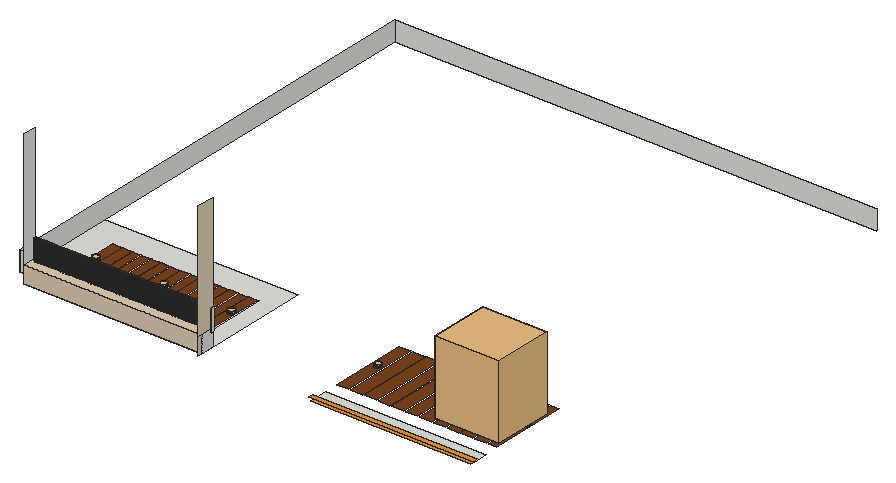
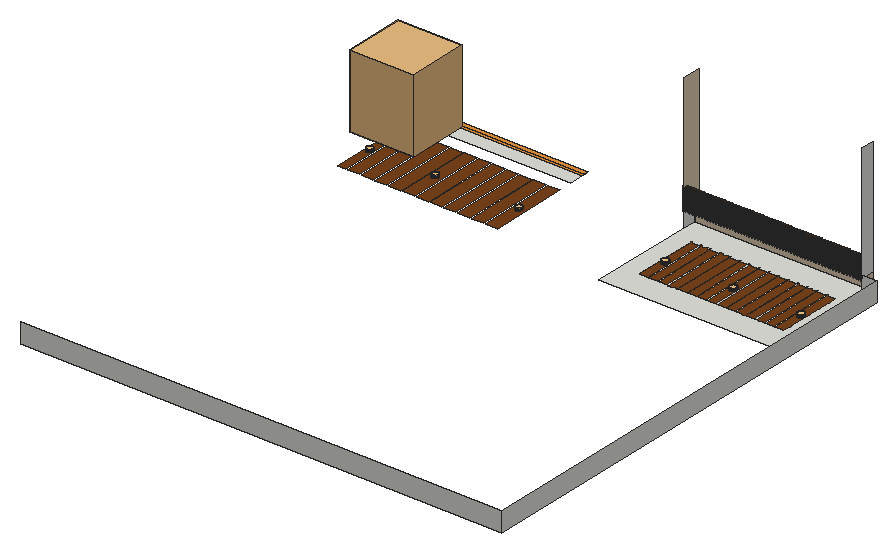
# SketchUp Ruby script. Lengths in inches.
U = 1.inch
M = Sketchup.active_model
def pt(a) = Geom::Point3d.new(a.map { |v| v * U })
def face(e, loops, mat)
  f = e.add_face(loops[0].map { |a| pt(a) })
  loops[1..].each { |l| e.add_face(l.map { |a| pt(a) }).erase! }
  f.material = f.back_material = mat if mat
  f
end
# faces: each face lists its corners as indices into pts; further lists are holes
def faces(e, pts, list, mat = nil) = list.each { |f| face(e, (f[0].is_a?(Array) ? f : [f]).map { |l| l.map { |i| pts[i] } }, mat) }
# xy, xz, yz: faces in a plane at the given z, y or x. An outline is a flat list of corners, or four numbers for a rectangle; further outlines are holes
def ring(l) = l.size == 4 ? [[l[0], l[1]], [l[2], l[1]], [l[2], l[3]], [l[0], l[3]]] : l.each_slice(2).to_a
def flat(e, list, mat, &to3) = list.each { |f| face(e, (f[0].is_a?(Array) ? f : [f]).map { |l| ring(l).map { |u, v| to3.(u, v) } }, mat) }
def xy(e, z, list, mat = nil) = flat(e, list, mat) { |x, y| [x, y, z] }
def xz(e, y, list, mat = nil) = flat(e, list, mat) { |x, z| [x, y, z] }
def yz(e, x, list, mat = nil) = flat(e, list, mat) { |y, z| [x, y, z] }
def lines(e, pts, list) = list.each { |a, b| e.add_line(pt(pts[a]), pt(pts[b])) }
# prism: a flat outline (further loops are holes) pulled along v
def prism(e, loops, v, mat = nil)
  f = face(e, loops, mat); d = Geom::Vector3d.new(v.map { |x| x * U })
  f.pushpull(f.normal.samedirection?(d) ? d.length : -d.length)
end
def box(e, o, s, mat = nil) = prism(e, [[o, [o[0] + s[0], o[1], o[2]], [o[0] + s[0], o[1] + s[1], o[2]], [o[0], o[1] + s[1], o[2]]]], [0, 0, s[2]], mat)
def at(x, y, z, deg = 0) = Geom::Transformation.translation(pt([x, y, z])) * Geom::Transformation.rotation(ORIGIN, Z_AXIS, deg.degrees)
def axes(o, x, y, z) = Geom::Transformation.new([*x, 0, *y, 0, *z, 0, *pt(o).to_a, 1])
def part(name) = M.definitions.add(name)
# library, detail: a bought-in or finely detailed component or shape, given as its bounding box
def library(name, o, s) = part(name).tap { |d| box(d.entities, o, s) }
def detail(e, o, s) = box(e.add_group.entities, o, s)
def put(e, d, t, mat = nil) = e.add_instance(d, t).tap { |i| i.material = mat if mat }
def group(e, t, mat = nil) = e.add_group.tap { |g| g.transformation = t; g.material = mat if mat }.entities
root = M.entities
M.materials.add("Generic\#1").color = [121, 68, 27]
M.materials.add("Generic\#2").color = [245, 199, 133]
M.materials.add("Generic\#4").color = [232, 149, 60]
M.materials.add("Generic\#6").color = [223, 205, 179]
c1 = library("Flora+17",[-57.52,158.6,-38.64],[66.99,62.88,77.28])
c2 = part("Group\#9")
xy(c2.entities,22.76,[[0,0,2,3]])
xz(c2.entities,0,[[0,0,2,22.76]])
yz(c2.entities,0,[[0,0,3,22.76]])
yz(c2.entities,2,[[0,0,3,22.76]])
xy(root,401.75,[[323.78,39.375,491.8125,54.5625],[[17.125,41,204.09,41,204.09,166.1875,2.3125,166.1875,2.3125,54.5625,17.125,54.5625],[32.72,68.9375,185.53,138.25]],[41.97,68.9375,42.91,138.25],[52.16,68.9375,53.09,138.25],[62.34,68.9375,63.28,138.25],
  [72.53,68.9375,73.47,138.25],[82.72,68.9375,83.66,138.25],[92.91,68.9375,93.84,138.25],[103.09,68.9375,104.03,138.25],[113.28,68.9375,114.22,138.25],
  [123.47,68.9375,124.41,138.25],[133.66,68.9375,134.59,138.25],[143.84,68.9375,144.78,138.25],[154.03,68.9375,154.97,138.25],[164.22,68.9375,165.16,138.25],
  [174.41,68.9375,175.34,138.25],[184.59,68.9375,185.53,138.25]])
xy(root,401.75,[[[32.72,68.9375,41.97,138.25],[37.48,106.29,38.4,106.47,39.23,106.87,39.93,107.48,40.46,108.25,40.76,109.13,40.83,110.06,40.65,110.97,40.24,111.81,39.63,112.51,38.86,113.03,37.98,113.34,37.06,113.4,36.14,113.23,35.31,112.82,34.6,112.21,34.08,111.44,33.78,110.5625,33.71,109.63,33.89,108.72,34.3,107.88,34.91,107.18,35.68,106.66,36.55,106.36]],[42.91,68.9375,52.16,138.25],[53.09,68.9375,62.34,138.25],[63.28,68.9375,72.53,138.25],[73.47,68.9375,82.72,138.25],
  [83.66,68.9375,92.91,138.25],[93.84,68.9375,103.09,138.25],[[104.03,68.9375,113.28,138.25],[108.73,106.29,109.65,106.47,110.48,106.87,111.18,107.48,111.71,108.25,112.01,109.13,112.08,110.06,111.9,110.97,111.49,111.81,110.88,112.51,110.11,113.03,109.23,113.34,108.31,113.4,107.39,113.23,106.56,112.82,105.85,112.21,105.33,111.44,105.03,110.5625,104.96,109.63,105.14,108.72,105.55,107.88,106.16,107.18,106.93,106.66,107.8,106.36]],[114.22,68.9375,123.47,138.25],[124.41,68.9375,133.66,138.25],
  [134.59,68.9375,143.84,138.25],[144.78,68.9375,154.03,138.25],[154.97,68.9375,164.22,138.25],[165.16,68.9375,174.41,138.25],[[175.34,68.9375,184.59,138.25],[180.17,106.29,181.08,106.47,181.92,106.87,182.62,107.48,183.14,108.25,183.45,109.13,183.51,110.06,183.34,110.97,182.93,111.81,182.32,112.51,181.55,113.03,180.67,113.34,179.74,113.4,178.83,113.23,177.99,112.82,177.29,112.21,176.77,111.44,176.47,110.5625,176.4,109.63,176.58,108.72,176.98,107.88,177.59,107.18,178.36,106.66,179.24,106.36]],
  [[323.03,69.49,335.53,151.25],[329.74,111.47,330.6,111.58,331.4,111.91,332.08,112.4375,332.61,113.125,332.94,113.92,333.05,114.78,332.94,115.64,332.61,116.4375,332.08,117.12,331.4,117.65,330.6,117.98,329.74,118.09,328.88,117.98,328.08,117.65,327.4,117.12,326.87,116.4375,326.54,115.64,326.43,114.78,326.54,113.92,326.87,113.125,327.4,112.4375,328.08,111.91,328.88,111.58]],[337.53,69.49,350.03,151.25],[352.03,69.49,364.53,151.25],[366.53,69.49,379.03,151.25],[381.03,69.49,393.53,151.25],
  [395.53,69.49,408.03,151.25],[[410.03,69.49,422.53,151.25],[417.49,111.47,418.35,111.58,419.15,111.91,419.83,112.4375,420.36,113.125,420.69,113.92,420.8,114.78,420.69,115.64,420.36,116.4375,419.83,117.12,419.15,117.65,418.35,117.98,417.49,118.09,416.63,117.98,415.83,117.65,415.15,117.12,414.62,116.4375,414.29,115.64,414.18,114.78,414.29,113.92,414.62,113.125,415.15,112.4375,415.83,111.91,416.63,111.58]],[424.53,69.49,437.03,151.25],[439.03,69.49,451.53,151.25],[453.53,69.49,466.03,151.25],
  [468.03,69.49,480.53,151.25],[[482.53,69.49,490.94,151.25],[486.8,111.47,487.66,111.58,488.46,111.91,489.15,112.4375,489.67,113.125,490,113.92,490.12,114.78,490,115.64,489.67,116.4375,489.15,117.12,488.46,117.65,487.66,117.98,486.8,118.09,485.95,117.98,485.15,117.65,484.46,117.12,483.93,116.4375,483.6,115.64,483.49,114.78,483.6,113.92,483.93,113.125,484.46,112.4375,485.15,111.91,485.95,111.58]]],"Generic\#1")
xy(root,401.75,[[323.78,34.75,491.8125,39.375]],"Generic\#4")
xy(root,404.3125,[[37.48,106.29,36.55,106.36,35.68,106.66,34.91,107.18,34.3,107.88,33.89,108.72,33.71,109.63,33.78,110.5625,34.08,111.44,34.6,112.21,35.31,112.82,36.14,113.23,37.06,113.4,37.98,113.34,38.86,113.03,39.63,112.51,40.24,111.81,40.65,110.97,40.83,110.06,40.76,109.13,40.46,108.25,39.93,107.48,39.23,106.87,38.4,106.47],[108.73,106.29,107.8,106.36,106.93,106.66,106.16,107.18,105.55,107.88,105.14,108.72,104.96,109.63,105.03,110.5625,105.33,111.44,105.85,112.21,106.56,112.82,107.39,113.23,108.31,113.4,109.23,113.34,110.11,113.03,110.88,112.51,111.49,111.81,111.9,110.97,112.08,110.06,112.01,109.13,111.71,108.25,111.18,107.48,110.48,106.87,109.65,106.47],[180.17,106.29,179.24,106.36,178.36,106.66,177.59,107.18,176.98,107.88,176.58,108.72,176.4,109.63,176.47,110.5625,176.77,111.44,177.29,112.21,177.99,112.82,178.83,113.23,179.74,113.4,180.67,113.34,181.55,113.03,182.32,112.51,182.93,111.81,183.34,110.97,183.51,110.06,183.45,109.13,183.14,108.25,182.62,107.48,181.92,106.87,181.08,106.47],[329.74,111.47,328.88,111.58,328.08,111.91,327.4,112.4375,326.87,113.125,326.54,113.92,326.43,114.78,326.54,115.64,326.87,116.4375,327.4,117.12,328.08,117.65,328.88,117.98,329.74,118.09,330.6,117.98,331.4,117.65,332.08,117.12,332.61,116.4375,332.94,115.64,333.05,114.78,332.94,113.92,332.61,113.125,332.08,112.4375,331.4,111.91,330.6,111.58],[417.49,111.47,416.63,111.58,415.83,111.91,415.15,112.4375,414.62,113.125,414.29,113.92,414.18,114.78,414.29,115.64,414.62,116.4375,415.15,117.12,415.83,117.65,416.63,117.98,417.49,118.09,418.35,117.98,419.15,117.65,419.83,117.12,420.36,116.4375,420.69,115.64,420.8,114.78,420.69,113.92,420.36,113.125,419.83,112.4375,419.15,111.91,418.35,111.58],
  [486.8,111.47,485.95,111.58,485.15,111.91,484.46,112.4375,483.93,113.125,483.6,113.92,483.49,114.78,483.6,115.64,483.93,116.4375,484.46,117.12,485.15,117.65,485.95,117.98,486.8,118.09,487.66,117.98,488.46,117.65,489.15,117.12,489.67,116.4375,490,115.64,490.12,114.78,490,113.92,489.67,113.125,489.15,112.4375,488.46,111.91,487.66,111.58]],"Generic\#2")
xy(root,404.6875,[[321.31,34.75,494.1875,39.375]],"Generic\#4")
xy(root,419.625,[[17.125,41,204.09,54.5625]],"Generic\#6")
xz(root,41,[[17.125,401.75,204.09,419.625]],"Generic\#6")
xz(root,54.5625,[[2.3125,401.75,17.125,422.625],[17.125,419.625,204.09,440.1875]])
xz(root,546.8125,[[2.3125,401.75,507.875,422.625]])
yz(root,2.3125,[[54.5625,401.75,546.8125,422.625]])
yz(root,17.125,[[41,419.625,54.5625,542.625]])
yz(root,204.09,[[41,401.75,54.5625,419.625]])
yz(root,204.09,[[35.5625,401.75,41,419.625],[35.5625,419.625,54.5625,542.625]],"Generic\#6")
p = [[37.48,106.29,401.75],[36.55,106.36,401.75],[36.55,106.36,404.3125],[37.48,106.29,404.3125],[38.4,106.47,401.75],[38.4,106.47,404.3125],
  [108.73,106.29,401.75],[107.8,106.36,401.75],[107.8,106.36,404.3125],[108.73,106.29,404.3125],[109.65,106.47,401.75],[109.65,106.47,404.3125],
  [180.17,106.29,401.75],[179.24,106.36,401.75],[179.24,106.36,404.3125],[180.17,106.29,404.3125],[181.08,106.47,401.75],[181.08,106.47,404.3125],
  [35.68,106.66,401.75],[35.68,106.66,404.3125],[106.93,106.66,401.75],[106.93,106.66,404.3125],[178.36,106.66,401.75],[178.36,106.66,404.3125],
  [39.23,106.87,401.75],[39.23,106.87,404.3125],[110.48,106.87,401.75],[110.48,106.87,404.3125],[181.92,106.87,401.75],[181.92,106.87,404.3125],
  [34.91,107.18,401.75],[34.91,107.18,404.3125],[106.16,107.18,401.75],[106.16,107.18,404.3125],[177.59,107.18,401.75],[177.59,107.18,404.3125],
  [39.93,107.48,401.75],[39.93,107.48,404.3125],[111.18,107.48,401.75],[111.18,107.48,404.3125],[182.62,107.48,401.75],[182.62,107.48,404.3125],
  [34.3,107.88,401.75],[34.3,107.88,404.3125],[105.55,107.88,401.75],[105.55,107.88,404.3125],[176.98,107.88,401.75],[176.98,107.88,404.3125],
  [40.46,108.25,401.75],[40.46,108.25,404.3125],[111.71,108.25,401.75],[111.71,108.25,404.3125],[183.14,108.25,401.75],[183.14,108.25,404.3125],
  [33.89,108.72,401.75],[33.89,108.72,404.3125],[105.14,108.72,401.75],[105.14,108.72,404.3125],[176.58,108.72,401.75],[176.58,108.72,404.3125],
  [40.76,109.13,401.75],[40.76,109.13,404.3125],[112.01,109.13,401.75],[112.01,109.13,404.3125],[183.45,109.13,401.75],[183.45,109.13,404.3125],
  [33.71,109.63,401.75],[33.71,109.63,404.3125],[104.96,109.63,401.75],[104.96,109.63,404.3125],[176.4,109.63,401.75],[176.4,109.63,404.3125],
  [40.83,110.06,401.75],[40.83,110.06,404.3125],[112.08,110.06,401.75],[112.08,110.06,404.3125],[183.51,110.06,401.75],[183.51,110.06,404.3125],
  [33.78,110.5625,401.75],[33.78,110.5625,404.3125],[105.03,110.5625,401.75],[105.03,110.5625,404.3125],[176.47,110.5625,401.75],[176.47,110.5625,404.3125],
  [40.65,110.97,401.75],[40.65,110.97,404.3125],[111.9,110.97,401.75],[111.9,110.97,404.3125],[183.34,110.97,401.75],[183.34,110.97,404.3125],
  [34.08,111.44,401.75],[34.08,111.44,404.3125],[105.33,111.44,401.75],[105.33,111.44,404.3125],[176.77,111.44,401.75],[176.77,111.44,404.3125],
  [40.24,111.81,401.75],[40.24,111.81,404.3125],[111.49,111.81,401.75],[111.49,111.81,404.3125],[182.93,111.81,401.75],[182.93,111.81,404.3125],
  [34.6,112.21,401.75],[34.6,112.21,404.3125],[105.85,112.21,401.75],[105.85,112.21,404.3125],[177.29,112.21,401.75],[177.29,112.21,404.3125],
  [329.74,111.47,401.75],[328.88,111.58,401.75],[328.88,111.58,404.3125],[329.74,111.47,404.3125],[330.6,111.58,401.75],[330.6,111.58,404.3125],
  [417.49,111.47,401.75],[416.63,111.58,401.75],[416.63,111.58,404.3125],[417.49,111.47,404.3125],[418.35,111.58,401.75],[418.35,111.58,404.3125],
  [486.8,111.47,401.75],[485.95,111.58,401.75],[485.95,111.58,404.3125],[486.8,111.47,404.3125],[487.66,111.58,401.75],[487.66,111.58,404.3125],
  [328.08,111.91,401.75],[328.08,111.91,404.3125],[331.4,111.91,401.75],[331.4,111.91,404.3125],[415.83,111.91,401.75],[415.83,111.91,404.3125],
  [419.15,111.91,401.75],[419.15,111.91,404.3125],[485.15,111.91,401.75],[485.15,111.91,404.3125],[488.46,111.91,401.75],[488.46,111.91,404.3125],
  [39.63,112.51,401.75],[39.63,112.51,404.3125],[110.88,112.51,401.75],[110.88,112.51,404.3125],[182.32,112.51,401.75],[182.32,112.51,404.3125],
  [327.4,112.4375,401.75],[327.4,112.4375,404.3125],[332.08,112.4375,401.75],[332.08,112.4375,404.3125],[415.15,112.4375,401.75],[415.15,112.4375,404.3125],
  [419.83,112.4375,401.75],[419.83,112.4375,404.3125],[484.46,112.4375,401.75],[484.46,112.4375,404.3125],[489.15,112.4375,401.75],[489.15,112.4375,404.3125],
  [35.31,112.82,401.75],[35.31,112.82,404.3125],[106.56,112.82,401.75],[106.56,112.82,404.3125],[177.99,112.82,401.75],[177.99,112.82,404.3125],
  [326.87,113.125,401.75],[326.87,113.125,404.3125],[332.61,113.125,401.75],[332.61,113.125,404.3125],[414.62,113.125,401.75],[414.62,113.125,404.3125],
  [420.36,113.125,401.75],[420.36,113.125,404.3125],[483.93,113.125,401.75],[483.93,113.125,404.3125],[489.67,113.125,401.75],[489.67,113.125,404.3125],
  [38.86,113.03,401.75],[38.86,113.03,404.3125],[110.11,113.03,401.75],[110.11,113.03,404.3125],[181.55,113.03,401.75],[181.55,113.03,404.3125],
  [36.14,113.23,401.75],[36.14,113.23,404.3125],[107.39,113.23,401.75],[107.39,113.23,404.3125],[178.83,113.23,401.75],[178.83,113.23,404.3125],
  [37.98,113.34,401.75],[37.98,113.34,404.3125],[109.23,113.34,401.75],[109.23,113.34,404.3125],[180.67,113.34,401.75],[180.67,113.34,404.3125],
  [326.54,113.92,401.75],[326.54,113.92,404.3125],[332.94,113.92,401.75],[332.94,113.92,404.3125],[414.29,113.92,401.75],[414.29,113.92,404.3125],
  [420.69,113.92,401.75],[420.69,113.92,404.3125],[483.6,113.92,401.75],[483.6,113.92,404.3125],[490,113.92,401.75],[490,113.92,404.3125],
  [37.06,113.4,401.75],[37.06,113.4,404.3125],[108.31,113.4,401.75],[108.31,113.4,404.3125],[179.74,113.4,401.75],[179.74,113.4,404.3125],
  [326.43,114.78,401.75],[326.43,114.78,404.3125],[333.05,114.78,401.75],[333.05,114.78,404.3125],[414.18,114.78,401.75],[414.18,114.78,404.3125],
  [420.8,114.78,401.75],[420.8,114.78,404.3125],[483.49,114.78,401.75],[483.49,114.78,404.3125],[490.12,114.78,401.75],[490.12,114.78,404.3125],
  [326.54,115.64,401.75],[326.54,115.64,404.3125],[332.94,115.64,401.75],[332.94,115.64,404.3125],[414.29,115.64,401.75],[414.29,115.64,404.3125],
  [420.69,115.64,401.75],[420.69,115.64,404.3125],[483.6,115.64,401.75],[483.6,115.64,404.3125],[490,115.64,401.75],[490,115.64,404.3125],
  [326.87,116.4375,401.75],[326.87,116.4375,404.3125],[332.61,116.4375,401.75],[332.61,116.4375,404.3125],[414.62,116.4375,401.75],[414.62,116.4375,404.3125],
  [420.36,116.4375,401.75],[420.36,116.4375,404.3125],[483.93,116.4375,401.75],[483.93,116.4375,404.3125],[489.67,116.4375,401.75],[489.67,116.4375,404.3125],
  [327.4,117.12,401.75],[327.4,117.12,404.3125],[332.08,117.12,401.75],[332.08,117.12,404.3125],[415.15,117.12,401.75],[415.15,117.12,404.3125],
  [419.83,117.12,401.75],[419.83,117.12,404.3125],[484.46,117.12,401.75],[484.46,117.12,404.3125],[489.15,117.12,401.75],[489.15,117.12,404.3125],
  [328.08,117.65,401.75],[328.08,117.65,404.3125],[331.4,117.65,401.75],[331.4,117.65,404.3125],[415.83,117.65,401.75],[415.83,117.65,404.3125],
  [419.15,117.65,401.75],[419.15,117.65,404.3125],[485.15,117.65,401.75],[485.15,117.65,404.3125],[488.46,117.65,401.75],[488.46,117.65,404.3125],
  [328.88,117.98,401.75],[328.88,117.98,404.3125],[330.6,117.98,401.75],[330.6,117.98,404.3125],[416.63,117.98,401.75],[416.63,117.98,404.3125],
  [418.35,117.98,401.75],[418.35,117.98,404.3125],[485.95,117.98,401.75],[485.95,117.98,404.3125],[487.66,117.98,401.75],[487.66,117.98,404.3125],
  [329.74,118.09,401.75],[329.74,118.09,404.3125],[417.49,118.09,401.75],[417.49,118.09,404.3125],[486.8,118.09,401.75],[486.8,118.09,404.3125],
  [32.72,68.9375,401.75],[31.78,68.9375,401.75],[31.78,138.25,401.75],[30.25,68.9375,401.75],[323.78,39.375,404.6875],[323.78,39.375,401.75]]
faces(root,p,[[0,1,2,3],[4,0,3,5],[6,7,8,9],[10,6,9,11],[12,13,14,15],[16,12,15,17],[1,18,19,2],[7,20,21,8],
  [13,22,23,14],[24,4,5,25],[26,10,11,27],[28,16,17,29],[18,30,31,19],[20,32,33,21],[22,34,35,23],[36,24,25,37],
  [38,26,27,39],[40,28,29,41],[30,42,43,31],[32,44,45,33],[34,46,47,35],[48,36,37,49],[50,38,39,51],[52,40,41,53],
  [42,54,55,43],[44,56,57,45],[46,58,59,47],[60,48,49,61],[62,50,51,63],[64,52,53,65],[54,66,67,55],[56,68,69,57],
  [58,70,71,59],[72,60,61,73],[74,62,63,75],[76,64,65,77],[66,78,79,67],[68,80,81,69],[70,82,83,71],[84,72,73,85],
  [86,74,75,87],[88,76,77,89],[78,90,91,79],[80,92,93,81],[82,94,95,83],[96,84,85,97],[98,86,87,99],[100,88,89,101],
  [90,102,103,91],[92,104,105,93],[94,106,107,95],[108,109,110,111],[112,108,111,113],[114,115,116,117],[118,114,117,119],[120,121,122,123],
  [124,120,123,125],[109,126,127,110],[128,112,113,129],[115,130,131,116],[132,118,119,133],[121,134,135,122],[136,124,125,137],[138,96,97,139],
  [140,98,99,141],[142,100,101,143],[126,144,145,127],[146,128,129,147],[130,148,149,131],[150,132,133,151],[134,152,153,135],[154,136,137,155],
  [102,156,157,103],[104,158,159,105],[106,160,161,107],[144,162,163,145],[164,146,147,165],[148,166,167,149],[168,150,151,169],[152,170,171,153],
  [172,154,155,173],[174,138,139,175],[176,140,141,177],[178,142,143,179],[156,180,181,157],[158,182,183,159],[160,184,185,161],[186,174,175,187],
  [188,176,177,189],[190,178,179,191],[162,192,193,163],[194,164,165,195],[166,196,197,167],[198,168,169,199],[170,200,201,171],[202,172,173,203],
  [180,204,205,181],[182,206,207,183],[184,208,209,185],[204,186,187,205],[206,188,189,207],[208,190,191,209],[192,210,211,193],[212,194,195,213],
  [196,214,215,197],[216,198,199,217],[200,218,219,201],[220,202,203,221],[210,222,223,211],[224,212,213,225],[214,226,227,215],[228,216,217,229],
  [218,230,231,219],[232,220,221,233],[222,234,235,223],[236,224,225,237],[226,238,239,227],[240,228,229,241],[230,242,243,231],[244,232,233,245],
  [234,246,247,235],[248,236,237,249],[238,250,251,239],[252,240,241,253],[242,254,255,243],[256,244,245,257],[246,258,259,247],[260,248,249,261],
  [250,262,263,251],[264,252,253,265],[254,266,267,255],[268,256,257,269],[258,270,271,259],[272,260,261,273],[262,274,275,263],[276,264,265,277],
  [266,278,279,267],[280,268,269,281],[270,282,283,271],[282,272,273,283],[274,284,285,275],[284,276,277,285],[278,286,287,279],[286,280,281,287]],"Generic\#2")
lines(root,p,[[288,289],[290,289],[289,291],[292,293]])
put(root,c1,at(493.76,-102.17,454.31))
put(root,c2,at(18.375,51.5625,417.43),"Generic\#1")
put(root,c2,at(21.3125,51.5625,417.43),"Generic\#1")
put(root,c2,at(24.25,51.5625,417.43),"Generic\#1")
put(root,c2,at(27.1875,51.5625,417.43),"Generic\#1")
put(root,c2,at(30.125,51.5625,417.43),"Generic\#1")
put(root,c2,at(33.0625,51.5625,417.43),"Generic\#1")
put(root,c2,at(36,51.5625,417.43),"Generic\#1")
put(root,c2,at(38.9375,51.5625,417.43),"Generic\#1")
put(root,c2,at(41.875,51.5625,417.43),"Generic\#1")
put(root,c2,at(44.8125,51.5625,417.43),"Generic\#1")
put(root,c2,at(47.75,51.5625,417.43),"Generic\#1")
put(root,c2,at(50.6875,51.5625,417.43),"Generic\#1")
put(root,c2,at(53.625,51.5625,417.43),"Generic\#1")
put(root,c2,at(56.5625,51.5625,417.43),"Generic\#1")
put(root,c2,at(59.5,51.5625,417.43),"Generic\#1")
put(root,c2,at(62.4375,51.5625,417.43),"Generic\#1")
put(root,c2,at(65.375,51.5625,417.43),"Generic\#1")
put(root,c2,at(68.3125,51.5625,417.43),"Generic\#1")
put(root,c2,at(71.25,51.5625,417.43),"Generic\#1")
put(root,c2,at(74.1875,51.5625,417.43),"Generic\#1")
put(root,c2,at(77.125,51.5625,417.43),"Generic\#1")
put(root,c2,at(80.0625,51.5625,417.43),"Generic\#1")
put(root,c2,at(83,51.5625,417.43),"Generic\#1")
put(root,c2,at(85.9375,51.5625,417.43),"Generic\#1")
put(root,c2,at(88.875,51.5625,417.43),"Generic\#1")
put(root,c2,at(91.8125,51.5625,417.43),"Generic\#1")
put(root,c2,at(94.75,51.5625,417.43),"Generic\#1")
put(root,c2,at(97.6875,51.5625,417.43),"Generic\#1")
put(root,c2,at(100.625,51.5625,417.43),"Generic\#1")
put(root,c2,at(103.5625,51.5625,417.43),"Generic\#1")
put(root,c2,at(106.5,51.5625,417.43),"Generic\#1")
put(root,c2,at(109.4375,51.5625,417.43),"Generic\#1")
put(root,c2,at(112.375,51.5625,417.43),"Generic\#1")
put(root,c2,at(115.3125,51.5625,417.43),"Generic\#1")
put(root,c2,at(118.25,51.5625,417.43),"Generic\#1")
put(root,c2,at(121.1875,51.5625,417.43),"Generic\#1")
put(root,c2,at(124.125,51.5625,417.43),"Generic\#1")
put(root,c2,at(127.0625,51.5625,417.43),"Generic\#1")
put(root,c2,at(130,51.5625,417.43),"Generic\#1")
put(root,c2,at(132.9375,51.5625,417.43),"Generic\#1")
put(root,c2,at(135.875,51.5625,417.43),"Generic\#1")
put(root,c2,at(138.8125,51.5625,417.43),"Generic\#1")
put(root,c2,at(141.75,51.5625,417.43),"Generic\#1")
put(root,c2,at(144.6875,51.5625,417.43),"Generic\#1")
put(root,c2,at(147.625,51.5625,417.43),"Generic\#1")
put(root,c2,at(150.5625,51.5625,417.43),"Generic\#1")
put(root,c2,at(153.5,51.5625,417.43),"Generic\#1")
put(root,c2,at(156.4375,51.5625,417.43),"Generic\#1")
put(root,c2,at(159.375,51.5625,417.43),"Generic\#1")
put(root,c2,at(162.3125,51.5625,417.43),"Generic\#1")
put(root,c2,at(165.25,51.5625,417.43),"Generic\#1")
put(root,c2,at(168.1875,51.5625,417.43),"Generic\#1")
put(root,c2,at(171.125,51.5625,417.43),"Generic\#1")
put(root,c2,at(174.0625,51.5625,417.43),"Generic\#1")
put(root,c2,at(177,51.5625,417.43),"Generic\#1")
put(root,c2,at(179.9375,51.5625,417.43),"Generic\#1")
put(root,c2,at(182.875,51.5625,417.43),"Generic\#1")
put(root,c2,at(185.8125,51.5625,417.43),"Generic\#1")
put(root,c2,at(188.75,51.5625,417.43),"Generic\#1")
put(root,c2,at(191.6875,51.5625,417.43),"Generic\#1")
put(root,c2,at(194.625,51.5625,417.43),"Generic\#1")
put(root,c2,at(197.75,51.5625,417.43),"Generic\#1")
put(root,c2,at(200.875,51.5625,417.43),"Generic\#1")
put(root,c2,at(204,51.5625,417.43))
